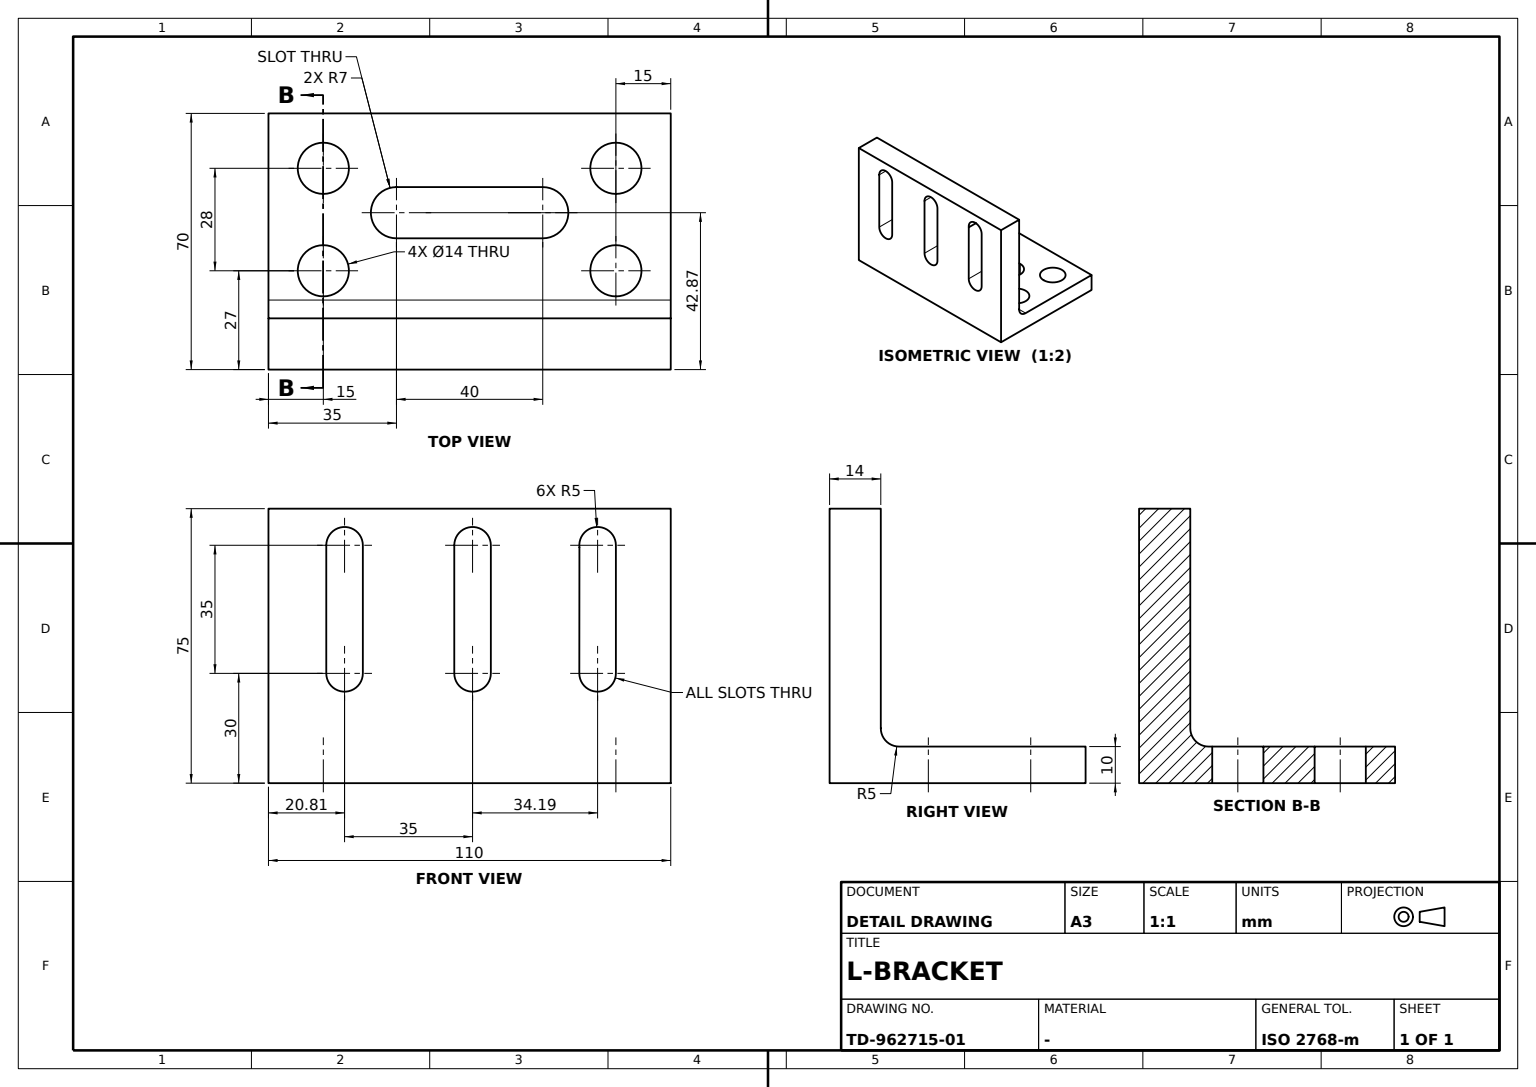
ISO-10303-21;
HEADER;
FILE_DESCRIPTION((''),'2;1');
FILE_NAME('','',(''),(''),'','','');
FILE_SCHEMA(('AUTOMOTIVE_DESIGN'));
ENDSEC;
DATA;
#1=APPLICATION_CONTEXT('');
#2=PRODUCT_CONTEXT('',#1,'mechanical');
#3=PRODUCT('','','',(#2));
#4=PRODUCT_DEFINITION_FORMATION('','',#3);
#5=PRODUCT_DEFINITION_CONTEXT('',#1,'design');
#6=PRODUCT_DEFINITION('','',#4,#5);
#7=PRODUCT_DEFINITION_SHAPE('','',#6);
#8=(LENGTH_UNIT()NAMED_UNIT(*)SI_UNIT(.MILLI.,.METRE.));
#9=(NAMED_UNIT(*)PLANE_ANGLE_UNIT()SI_UNIT($,.RADIAN.));
#10=(NAMED_UNIT(*)SI_UNIT($,.STERADIAN.)SOLID_ANGLE_UNIT());
#11=UNCERTAINTY_MEASURE_WITH_UNIT(LENGTH_MEASURE(0.005),#8,'distance_accuracy_value','');
#12=(GEOMETRIC_REPRESENTATION_CONTEXT(3)GLOBAL_UNCERTAINTY_ASSIGNED_CONTEXT((#11))GLOBAL_UNIT_ASSIGNED_CONTEXT((#8,#9,#10))REPRESENTATION_CONTEXT('',''));
#13=CARTESIAN_POINT('',(-7.,-24.969351,44.348961));
#14=VERTEX_POINT('',#13);
#15=CARTESIAN_POINT('',(7.,-24.969351,44.348961));
#16=VERTEX_POINT('',#15);
#17=DIRECTION('',(-1.,0.,0.));
#18=VECTOR('',#17,1000.);
#19=LINE('',#13,#18);
#20=EDGE_CURVE('',#14,#16,#19,.F.);
#21=ORIENTED_EDGE('',*,*,#20,.T.);
#22=CARTESIAN_POINT('',(7.,-24.999998,9.906179));
#23=VERTEX_POINT('',#22);
#24=CARTESIAN_POINT('',(7.,-25.026676,-20.076002));
#25=DIRECTION('',(0.,-0.000889801,-0.999999604));
#26=VECTOR('',#25,1000.);
#27=LINE('',#24,#26);
#28=EDGE_CURVE('',#16,#23,#27,.T.);
#29=ORIENTED_EDGE('',*,*,#28,.T.);
#30=CARTESIAN_POINT('',(-7.,-24.999998,9.906179));
#31=VERTEX_POINT('',#30);
#32=CARTESIAN_POINT('',(0.66,-24.999998,9.906179));
#33=LINE('',#32,#18);
#34=EDGE_CURVE('',#31,#23,#33,.F.);
#35=ORIENTED_EDGE('',*,*,#34,.F.);
#36=LINE('',#13,#26);
#37=EDGE_CURVE('',#14,#31,#36,.T.);
#38=ORIENTED_EDGE('',*,*,#37,.F.);
#39=EDGE_LOOP('',(#21,#29,#35,#38));
#40=FACE_BOUND('',#39,.T.);
#41=DIRECTION('',(0.,-0.999999604,0.000889801));
#42=AXIS2_PLACEMENT_3D('',#13,#41,#25);
#43=PLANE('',#42);
#44=ADVANCED_FACE('',(#40),#43,.F.);
#45=CARTESIAN_POINT('',(-7.,-15.,9.90173));
#46=VERTEX_POINT('',#45);
#47=CARTESIAN_POINT('',(-7.,-20.,9.90173));
#48=DIRECTION('',(0.,0.,1.));
#49=AXIS2_PLACEMENT_3D('',#47,#17,#48);
#50=CIRCLE('',#49,5.);
#51=EDGE_CURVE('',#46,#31,#50,.T.);
#52=ORIENTED_EDGE('',*,*,#51,.T.);
#53=ORIENTED_EDGE('',*,*,#34,.T.);
#54=CARTESIAN_POINT('',(7.,-15.,9.90173));
#55=VERTEX_POINT('',#54);
#56=CARTESIAN_POINT('',(7.,-20.,9.90173));
#57=DIRECTION('',(1.,0.,0.));
#58=DIRECTION('',(0.,0.,-1.));
#59=AXIS2_PLACEMENT_3D('',#56,#57,#58);
#60=CIRCLE('',#59,5.);
#61=EDGE_CURVE('',#23,#55,#60,.T.);
#62=ORIENTED_EDGE('',*,*,#61,.T.);
#63=CARTESIAN_POINT('',(0.66,-15.,9.90173));
#64=LINE('',#63,#18);
#65=EDGE_CURVE('',#46,#55,#64,.F.);
#66=ORIENTED_EDGE('',*,*,#65,.F.);
#67=EDGE_LOOP('',(#52,#53,#62,#66));
#68=FACE_BOUND('',#67,.T.);
#69=CARTESIAN_POINT('',(0.66,-20.,9.90173));
#70=DIRECTION('',(0.,-1.,0.));
#71=AXIS2_PLACEMENT_3D('',#69,#17,#70);
#72=CYLINDRICAL_SURFACE('',#71,5.);
#73=ADVANCED_FACE('',(#68),#72,.F.);
#74=CARTESIAN_POINT('',(-28.867531,-35.,-20.09827));
#75=VERTEX_POINT('',#74);
#76=CARTESIAN_POINT('',(-28.867531,-75.,-20.09827));
#77=VERTEX_POINT('',#76);
#78=CARTESIAN_POINT('',(-28.867531,0.,-20.09827));
#79=VECTOR('',#70,1000.);
#80=LINE('',#78,#79);
#81=EDGE_CURVE('',#75,#77,#80,.T.);
#82=ORIENTED_EDGE('',*,*,#81,.T.);
#83=CARTESIAN_POINT('',(-28.867531,-75.,-10.09827));
#84=VERTEX_POINT('',#83);
#85=CARTESIAN_POINT('',(-28.867531,-75.,-15.75827));
#86=VECTOR('',#48,1000.);
#87=LINE('',#85,#86);
#88=EDGE_CURVE('',#84,#77,#87,.F.);
#89=ORIENTED_EDGE('',*,*,#88,.F.);
#90=CARTESIAN_POINT('',(-28.867531,-35.,-10.09827));
#91=VERTEX_POINT('',#90);
#92=LINE('',#90,#79);
#93=EDGE_CURVE('',#91,#84,#92,.T.);
#94=ORIENTED_EDGE('',*,*,#93,.F.);
#95=CARTESIAN_POINT('',(-28.867531,-35.,-15.75827));
#96=LINE('',#95,#86);
#97=EDGE_CURVE('',#91,#75,#96,.F.);
#98=ORIENTED_EDGE('',*,*,#97,.T.);
#99=EDGE_LOOP('',(#82,#89,#94,#98));
#100=FACE_BOUND('',#99,.T.);
#101=AXIS2_PLACEMENT_3D('',#90,#57,#70);
#102=PLANE('',#101);
#103=ADVANCED_FACE('',(#100),#102,.F.);
#104=CARTESIAN_POINT('',(7.,-15.,44.90173));
#105=VERTEX_POINT('',#104);
#106=CARTESIAN_POINT('',(7.,-20.,44.90173));
#107=AXIS2_PLACEMENT_3D('',#106,#57,#58);
#108=CIRCLE('',#107,5.);
#109=EDGE_CURVE('',#105,#16,#108,.T.);
#110=ORIENTED_EDGE('',*,*,#109,.T.);
#111=ORIENTED_EDGE('',*,*,#20,.F.);
#112=CARTESIAN_POINT('',(-7.,-15.,44.90173));
#113=VERTEX_POINT('',#112);
#114=CARTESIAN_POINT('',(-7.,-20.,44.90173));
#115=AXIS2_PLACEMENT_3D('',#114,#17,#48);
#116=CIRCLE('',#115,5.);
#117=EDGE_CURVE('',#14,#113,#116,.T.);
#118=ORIENTED_EDGE('',*,*,#117,.T.);
#119=CARTESIAN_POINT('',(0.66,-15.,44.90173));
#120=LINE('',#119,#18);
#121=EDGE_CURVE('',#113,#105,#120,.F.);
#122=ORIENTED_EDGE('',*,*,#121,.T.);
#123=EDGE_LOOP('',(#110,#111,#118,#122));
#124=FACE_BOUND('',#123,.T.);
#125=CARTESIAN_POINT('',(0.66,-20.,44.90173));
#126=AXIS2_PLACEMENT_3D('',#125,#17,#70);
#127=CYLINDRICAL_SURFACE('',#126,5.);
#128=ADVANCED_FACE('',(#124),#127,.F.);
#129=VECTOR('',#58,1000.);
#130=LINE('',#112,#129);
#131=EDGE_CURVE('',#113,#46,#130,.T.);
#132=ORIENTED_EDGE('',*,*,#131,.T.);
#133=ORIENTED_EDGE('',*,*,#65,.T.);
#134=CARTESIAN_POINT('',(7.,-15.,-20.09827));
#135=LINE('',#134,#129);
#136=EDGE_CURVE('',#105,#55,#135,.T.);
#137=ORIENTED_EDGE('',*,*,#136,.F.);
#138=ORIENTED_EDGE('',*,*,#121,.F.);
#139=EDGE_LOOP('',(#132,#133,#137,#138));
#140=FACE_BOUND('',#139,.T.);
#141=AXIS2_PLACEMENT_3D('',#112,#70,#58);
#142=PLANE('',#141);
#143=ADVANCED_FACE('',(#140),#142,.T.);
#144=CARTESIAN_POINT('',(-13.,-15.,-10.09827));
#145=VERTEX_POINT('',#144);
#146=CARTESIAN_POINT('',(-20.,-15.,-10.09827));
#147=AXIS2_PLACEMENT_3D('',#146,#48,#57);
#148=CIRCLE('',#147,7.);
#149=EDGE_CURVE('',#145,#145,#148,.T.);
#150=ORIENTED_EDGE('',*,*,#149,.T.);
#151=EDGE_LOOP('',(#150));
#152=FACE_BOUND('',#151,.T.);
#153=CARTESIAN_POINT('',(-27.,-15.,-20.09827));
#154=VERTEX_POINT('',#153);
#155=CARTESIAN_POINT('',(-20.,-15.,-20.09827));
#156=AXIS2_PLACEMENT_3D('',#155,#58,#17);
#157=CIRCLE('',#156,7.);
#158=EDGE_CURVE('',#154,#154,#157,.T.);
#159=ORIENTED_EDGE('',*,*,#158,.T.);
#160=EDGE_LOOP('',(#159));
#161=FACE_BOUND('',#160,.T.);
#162=CARTESIAN_POINT('',(-20.,-15.,-15.75827));
#163=AXIS2_PLACEMENT_3D('',#162,#48,#57);
#164=CYLINDRICAL_SURFACE('',#163,7.);
#165=ADVANCED_FACE('',(#152,#161),#164,.F.);
#166=CARTESIAN_POINT('',(7.,-84.190727,44.90173));
#167=VERTEX_POINT('',#166);
#168=CARTESIAN_POINT('',(7.,-94.190727,44.90173));
#169=VERTEX_POINT('',#168);
#170=CARTESIAN_POINT('',(7.,-89.190727,44.90173));
#171=AXIS2_PLACEMENT_3D('',#170,#57,#58);
#172=CIRCLE('',#171,5.);
#173=EDGE_CURVE('',#167,#169,#172,.T.);
#174=ORIENTED_EDGE('',*,*,#173,.F.);
#175=CARTESIAN_POINT('',(7.,-84.190727,9.90173));
#176=VERTEX_POINT('',#175);
#177=CARTESIAN_POINT('',(7.,-84.190727,-20.09827));
#178=LINE('',#177,#129);
#179=EDGE_CURVE('',#167,#176,#178,.T.);
#180=ORIENTED_EDGE('',*,*,#179,.T.);
#181=CARTESIAN_POINT('',(7.,-94.190727,9.90173));
#182=VERTEX_POINT('',#181);
#183=CARTESIAN_POINT('',(7.,-89.190727,9.90173));
#184=AXIS2_PLACEMENT_3D('',#183,#57,#58);
#185=CIRCLE('',#184,5.);
#186=EDGE_CURVE('',#182,#176,#185,.T.);
#187=ORIENTED_EDGE('',*,*,#186,.F.);
#188=CARTESIAN_POINT('',(7.,-94.190727,-20.09827));
#189=LINE('',#188,#129);
#190=EDGE_CURVE('',#169,#182,#189,.T.);
#191=ORIENTED_EDGE('',*,*,#190,.F.);
#192=EDGE_LOOP('',(#174,#180,#187,#191));
#193=FACE_BOUND('',#192,.T.);
#194=ORIENTED_EDGE('',*,*,#61,.F.);
#195=ORIENTED_EDGE('',*,*,#28,.F.);
#196=ORIENTED_EDGE('',*,*,#109,.F.);
#197=ORIENTED_EDGE('',*,*,#136,.T.);
#198=EDGE_LOOP('',(#194,#195,#196,#197));
#199=FACE_BOUND('',#198,.T.);
#200=CARTESIAN_POINT('',(7.,-59.190727,44.90173));
#201=VERTEX_POINT('',#200);
#202=CARTESIAN_POINT('',(7.,-59.190727,9.90173));
#203=VERTEX_POINT('',#202);
#204=CARTESIAN_POINT('',(7.,-59.190727,-20.09827));
#205=LINE('',#204,#129);
#206=EDGE_CURVE('',#201,#203,#205,.T.);
#207=ORIENTED_EDGE('',*,*,#206,.F.);
#208=CARTESIAN_POINT('',(7.,-49.190727,44.90173));
#209=VERTEX_POINT('',#208);
#210=CARTESIAN_POINT('',(7.,-54.190727,44.90173));
#211=AXIS2_PLACEMENT_3D('',#210,#57,#58);
#212=CIRCLE('',#211,5.);
#213=EDGE_CURVE('',#209,#201,#212,.T.);
#214=ORIENTED_EDGE('',*,*,#213,.F.);
#215=CARTESIAN_POINT('',(7.,-49.190727,9.90173));
#216=VERTEX_POINT('',#215);
#217=CARTESIAN_POINT('',(7.,-49.190727,-20.09827));
#218=LINE('',#217,#129);
#219=EDGE_CURVE('',#209,#216,#218,.T.);
#220=ORIENTED_EDGE('',*,*,#219,.T.);
#221=CARTESIAN_POINT('',(7.,-54.190727,9.90173));
#222=AXIS2_PLACEMENT_3D('',#221,#57,#58);
#223=CIRCLE('',#222,5.);
#224=EDGE_CURVE('',#203,#216,#223,.T.);
#225=ORIENTED_EDGE('',*,*,#224,.F.);
#226=EDGE_LOOP('',(#207,#214,#220,#225));
#227=FACE_BOUND('',#226,.T.);
#228=CARTESIAN_POINT('',(7.,0.,54.90173));
#229=VERTEX_POINT('',#228);
#230=CARTESIAN_POINT('',(7.,-110.,54.90173));
#231=VERTEX_POINT('',#230);
#232=LINE('',#228,#79);
#233=EDGE_CURVE('',#229,#231,#232,.T.);
#234=ORIENTED_EDGE('',*,*,#233,.T.);
#235=CARTESIAN_POINT('',(7.,-110.,-20.09827));
#236=VERTEX_POINT('',#235);
#237=LINE('',#235,#86);
#238=EDGE_CURVE('',#236,#231,#237,.T.);
#239=ORIENTED_EDGE('',*,*,#238,.F.);
#240=CARTESIAN_POINT('',(7.,0.,-20.09827));
#241=VERTEX_POINT('',#240);
#242=LINE('',#240,#79);
#243=EDGE_CURVE('',#241,#236,#242,.T.);
#244=ORIENTED_EDGE('',*,*,#243,.F.);
#245=LINE('',#240,#86);
#246=EDGE_CURVE('',#241,#229,#245,.T.);
#247=ORIENTED_EDGE('',*,*,#246,.T.);
#248=EDGE_LOOP('',(#234,#239,#244,#247));
#249=FACE_BOUND('',#248,.T.);
#250=AXIS2_PLACEMENT_3D('',#240,#57,#48);
#251=PLANE('',#250);
#252=ADVANCED_FACE('',(#193,#199,#227,#249),#251,.T.);
#253=CARTESIAN_POINT('',(-7.,-84.190727,9.90173));
#254=VERTEX_POINT('',#253);
#255=CARTESIAN_POINT('',(0.66,-84.190727,9.90173));
#256=LINE('',#255,#18);
#257=EDGE_CURVE('',#254,#176,#256,.F.);
#258=ORIENTED_EDGE('',*,*,#257,.F.);
#259=CARTESIAN_POINT('',(-7.,-94.190727,9.90173));
#260=VERTEX_POINT('',#259);
#261=CARTESIAN_POINT('',(-7.,-89.190727,9.90173));
#262=AXIS2_PLACEMENT_3D('',#261,#17,#48);
#263=CIRCLE('',#262,5.);
#264=EDGE_CURVE('',#254,#260,#263,.T.);
#265=ORIENTED_EDGE('',*,*,#264,.T.);
#266=CARTESIAN_POINT('',(0.66,-94.190727,9.90173));
#267=LINE('',#266,#18);
#268=EDGE_CURVE('',#260,#182,#267,.F.);
#269=ORIENTED_EDGE('',*,*,#268,.T.);
#270=ORIENTED_EDGE('',*,*,#186,.T.);
#271=EDGE_LOOP('',(#258,#265,#269,#270));
#272=FACE_BOUND('',#271,.T.);
#273=CARTESIAN_POINT('',(0.66,-89.190727,9.90173));
#274=AXIS2_PLACEMENT_3D('',#273,#17,#70);
#275=CYLINDRICAL_SURFACE('',#274,5.);
#276=ADVANCED_FACE('',(#272),#275,.F.);
#277=CARTESIAN_POINT('',(-27.,-95.,-20.09827));
#278=VERTEX_POINT('',#277);
#279=CARTESIAN_POINT('',(-20.,-95.,-20.09827));
#280=AXIS2_PLACEMENT_3D('',#279,#58,#17);
#281=CIRCLE('',#280,7.);
#282=EDGE_CURVE('',#278,#278,#281,.T.);
#283=ORIENTED_EDGE('',*,*,#282,.F.);
#284=EDGE_LOOP('',(#283));
#285=FACE_BOUND('',#284,.T.);
#286=ORIENTED_EDGE('',*,*,#158,.F.);
#287=EDGE_LOOP('',(#286));
#288=FACE_BOUND('',#287,.T.);
#289=CARTESIAN_POINT('',(-63.,0.,-20.09827));
#290=VERTEX_POINT('',#289);
#291=CARTESIAN_POINT('',(-63.,-110.,-20.09827));
#292=VERTEX_POINT('',#291);
#293=LINE('',#289,#79);
#294=EDGE_CURVE('',#290,#292,#293,.T.);
#295=ORIENTED_EDGE('',*,*,#294,.F.);
#296=VECTOR('',#57,1000.);
#297=LINE('',#289,#296);
#298=EDGE_CURVE('',#290,#241,#297,.T.);
#299=ORIENTED_EDGE('',*,*,#298,.T.);
#300=ORIENTED_EDGE('',*,*,#243,.T.);
#301=LINE('',#291,#296);
#302=EDGE_CURVE('',#292,#236,#301,.T.);
#303=ORIENTED_EDGE('',*,*,#302,.F.);
#304=EDGE_LOOP('',(#295,#299,#300,#303));
#305=FACE_BOUND('',#304,.T.);
#306=CARTESIAN_POINT('',(-55.,-15.,-20.09827));
#307=VERTEX_POINT('',#306);
#308=CARTESIAN_POINT('',(-48.,-15.,-20.09827));
#309=AXIS2_PLACEMENT_3D('',#308,#58,#17);
#310=CIRCLE('',#309,7.);
#311=EDGE_CURVE('',#307,#307,#310,.T.);
#312=ORIENTED_EDGE('',*,*,#311,.F.);
#313=EDGE_LOOP('',(#312));
#314=FACE_BOUND('',#313,.T.);
#315=CARTESIAN_POINT('',(-42.867531,-75.,-20.09827));
#316=VERTEX_POINT('',#315);
#317=CARTESIAN_POINT('',(-35.867531,-75.,-20.09827));
#318=AXIS2_PLACEMENT_3D('',#317,#58,#17);
#319=CIRCLE('',#318,7.);
#320=EDGE_CURVE('',#77,#316,#319,.T.);
#321=ORIENTED_EDGE('',*,*,#320,.F.);
#322=ORIENTED_EDGE('',*,*,#81,.F.);
#323=CARTESIAN_POINT('',(-42.867531,-35.,-20.09827));
#324=VERTEX_POINT('',#323);
#325=CARTESIAN_POINT('',(-35.867531,-35.,-20.09827));
#326=AXIS2_PLACEMENT_3D('',#325,#58,#17);
#327=CIRCLE('',#326,7.);
#328=EDGE_CURVE('',#324,#75,#327,.T.);
#329=ORIENTED_EDGE('',*,*,#328,.F.);
#330=CARTESIAN_POINT('',(-42.867531,0.,-20.09827));
#331=LINE('',#330,#79);
#332=EDGE_CURVE('',#324,#316,#331,.T.);
#333=ORIENTED_EDGE('',*,*,#332,.T.);
#334=EDGE_LOOP('',(#321,#322,#329,#333));
#335=FACE_BOUND('',#334,.T.);
#336=CARTESIAN_POINT('',(-55.,-95.,-20.09827));
#337=VERTEX_POINT('',#336);
#338=CARTESIAN_POINT('',(-48.,-95.,-20.09827));
#339=AXIS2_PLACEMENT_3D('',#338,#58,#17);
#340=CIRCLE('',#339,7.);
#341=EDGE_CURVE('',#337,#337,#340,.T.);
#342=ORIENTED_EDGE('',*,*,#341,.F.);
#343=EDGE_LOOP('',(#342));
#344=FACE_BOUND('',#343,.T.);
#345=AXIS2_PLACEMENT_3D('',#289,#58,#57);
#346=PLANE('',#345);
#347=ADVANCED_FACE('',(#285,#288,#305,#314,#335,#344),#346,.T.);
#348=CARTESIAN_POINT('',(-42.867531,-35.,-10.09827));
#349=VERTEX_POINT('',#348);
#350=CARTESIAN_POINT('',(-42.867531,-35.,-15.75827));
#351=LINE('',#350,#86);
#352=EDGE_CURVE('',#349,#324,#351,.F.);
#353=ORIENTED_EDGE('',*,*,#352,.F.);
#354=CARTESIAN_POINT('',(-42.867531,-75.,-10.09827));
#355=VERTEX_POINT('',#354);
#356=LINE('',#348,#79);
#357=EDGE_CURVE('',#349,#355,#356,.T.);
#358=ORIENTED_EDGE('',*,*,#357,.T.);
#359=CARTESIAN_POINT('',(-42.867531,-75.,-15.75827));
#360=LINE('',#359,#86);
#361=EDGE_CURVE('',#355,#316,#360,.F.);
#362=ORIENTED_EDGE('',*,*,#361,.T.);
#363=ORIENTED_EDGE('',*,*,#332,.F.);
#364=EDGE_LOOP('',(#353,#358,#362,#363));
#365=FACE_BOUND('',#364,.T.);
#366=AXIS2_PLACEMENT_3D('',#348,#57,#70);
#367=PLANE('',#366);
#368=ADVANCED_FACE('',(#365),#367,.T.);
#369=ORIENTED_EDGE('',*,*,#233,.F.);
#370=CARTESIAN_POINT('',(-7.,0.,54.90173));
#371=VERTEX_POINT('',#370);
#372=LINE('',#228,#18);
#373=EDGE_CURVE('',#229,#371,#372,.T.);
#374=ORIENTED_EDGE('',*,*,#373,.T.);
#375=CARTESIAN_POINT('',(-7.,-110.,54.90173));
#376=VERTEX_POINT('',#375);
#377=LINE('',#370,#79);
#378=EDGE_CURVE('',#371,#376,#377,.T.);
#379=ORIENTED_EDGE('',*,*,#378,.T.);
#380=LINE('',#230,#18);
#381=EDGE_CURVE('',#231,#376,#380,.T.);
#382=ORIENTED_EDGE('',*,*,#381,.F.);
#383=EDGE_LOOP('',(#369,#374,#379,#382));
#384=FACE_BOUND('',#383,.T.);
#385=AXIS2_PLACEMENT_3D('',#228,#48,#17);
#386=PLANE('',#385);
#387=ADVANCED_FACE('',(#384),#386,.T.);
#388=CARTESIAN_POINT('',(-7.,-49.190727,9.90173));
#389=VERTEX_POINT('',#388);
#390=CARTESIAN_POINT('',(0.66,-49.190727,9.90173));
#391=LINE('',#390,#18);
#392=EDGE_CURVE('',#389,#216,#391,.F.);
#393=ORIENTED_EDGE('',*,*,#392,.T.);
#394=ORIENTED_EDGE('',*,*,#219,.F.);
#395=CARTESIAN_POINT('',(-7.,-49.190727,44.90173));
#396=VERTEX_POINT('',#395);
#397=CARTESIAN_POINT('',(0.66,-49.190727,44.90173));
#398=LINE('',#397,#18);
#399=EDGE_CURVE('',#396,#209,#398,.F.);
#400=ORIENTED_EDGE('',*,*,#399,.F.);
#401=LINE('',#395,#129);
#402=EDGE_CURVE('',#396,#389,#401,.T.);
#403=ORIENTED_EDGE('',*,*,#402,.T.);
#404=EDGE_LOOP('',(#393,#394,#400,#403));
#405=FACE_BOUND('',#404,.T.);
#406=AXIS2_PLACEMENT_3D('',#395,#70,#58);
#407=PLANE('',#406);
#408=ADVANCED_FACE('',(#405),#407,.T.);
#409=CARTESIAN_POINT('',(-7.,-59.190727,44.90173));
#410=VERTEX_POINT('',#409);
#411=CARTESIAN_POINT('',(0.66,-59.190727,44.90173));
#412=LINE('',#411,#18);
#413=EDGE_CURVE('',#410,#201,#412,.F.);
#414=ORIENTED_EDGE('',*,*,#413,.T.);
#415=ORIENTED_EDGE('',*,*,#206,.T.);
#416=CARTESIAN_POINT('',(-7.,-59.190727,9.90173));
#417=VERTEX_POINT('',#416);
#418=CARTESIAN_POINT('',(0.66,-59.190727,9.90173));
#419=LINE('',#418,#18);
#420=EDGE_CURVE('',#417,#203,#419,.F.);
#421=ORIENTED_EDGE('',*,*,#420,.F.);
#422=LINE('',#409,#129);
#423=EDGE_CURVE('',#410,#417,#422,.T.);
#424=ORIENTED_EDGE('',*,*,#423,.F.);
#425=EDGE_LOOP('',(#414,#415,#421,#424));
#426=FACE_BOUND('',#425,.T.);
#427=AXIS2_PLACEMENT_3D('',#409,#70,#58);
#428=PLANE('',#427);
#429=ADVANCED_FACE('',(#426),#428,.F.);
#430=ORIENTED_EDGE('',*,*,#341,.T.);
#431=EDGE_LOOP('',(#430));
#432=FACE_BOUND('',#431,.T.);
#433=CARTESIAN_POINT('',(-41.,-95.,-10.09827));
#434=VERTEX_POINT('',#433);
#435=CARTESIAN_POINT('',(-48.,-95.,-10.09827));
#436=AXIS2_PLACEMENT_3D('',#435,#48,#57);
#437=CIRCLE('',#436,7.);
#438=EDGE_CURVE('',#434,#434,#437,.T.);
#439=ORIENTED_EDGE('',*,*,#438,.T.);
#440=EDGE_LOOP('',(#439));
#441=FACE_BOUND('',#440,.T.);
#442=CARTESIAN_POINT('',(-48.,-95.,-15.75827));
#443=AXIS2_PLACEMENT_3D('',#442,#48,#57);
#444=CYLINDRICAL_SURFACE('',#443,7.);
#445=ADVANCED_FACE('',(#432,#441),#444,.F.);
#446=CARTESIAN_POINT('',(-35.867531,-75.,-10.09827));
#447=AXIS2_PLACEMENT_3D('',#446,#48,#57);
#448=CIRCLE('',#447,7.);
#449=EDGE_CURVE('',#355,#84,#448,.T.);
#450=ORIENTED_EDGE('',*,*,#449,.T.);
#451=ORIENTED_EDGE('',*,*,#88,.T.);
#452=ORIENTED_EDGE('',*,*,#320,.T.);
#453=ORIENTED_EDGE('',*,*,#361,.F.);
#454=EDGE_LOOP('',(#450,#451,#452,#453));
#455=FACE_BOUND('',#454,.T.);
#456=CARTESIAN_POINT('',(-35.867531,-75.,-15.75827));
#457=AXIS2_PLACEMENT_3D('',#456,#48,#57);
#458=CYLINDRICAL_SURFACE('',#457,7.);
#459=ADVANCED_FACE('',(#455),#458,.F.);
#460=ORIENTED_EDGE('',*,*,#246,.F.);
#461=ORIENTED_EDGE('',*,*,#298,.F.);
#462=CARTESIAN_POINT('',(-63.,0.,-10.09827));
#463=VERTEX_POINT('',#462);
#464=LINE('',#462,#129);
#465=EDGE_CURVE('',#463,#290,#464,.T.);
#466=ORIENTED_EDGE('',*,*,#465,.F.);
#467=CARTESIAN_POINT('',(-12.,0.,-10.09827));
#468=VERTEX_POINT('',#467);
#469=CARTESIAN_POINT('',(-7.,0.,-10.09827));
#470=LINE('',#469,#18);
#471=EDGE_CURVE('',#468,#463,#470,.T.);
#472=ORIENTED_EDGE('',*,*,#471,.F.);
#473=CARTESIAN_POINT('',(-7.,0.,-5.09827));
#474=VERTEX_POINT('',#473);
#475=CARTESIAN_POINT('',(-12.,0.,-5.09827));
#476=DIRECTION('',(0.,1.,0.));
#477=AXIS2_PLACEMENT_3D('',#475,#476,#48);
#478=CIRCLE('',#477,5.);
#479=EDGE_CURVE('',#474,#468,#478,.T.);
#480=ORIENTED_EDGE('',*,*,#479,.F.);
#481=LINE('',#370,#129);
#482=EDGE_CURVE('',#371,#474,#481,.T.);
#483=ORIENTED_EDGE('',*,*,#482,.F.);
#484=ORIENTED_EDGE('',*,*,#373,.F.);
#485=EDGE_LOOP('',(#460,#461,#466,#472,#480,#483,#484));
#486=FACE_BOUND('',#485,.T.);
#487=CARTESIAN_POINT('',(0.,0.,0.));
#488=AXIS2_PLACEMENT_3D('',#487,#476,#17);
#489=PLANE('',#488);
#490=ADVANCED_FACE('',(#486),#489,.T.);
#491=CARTESIAN_POINT('',(-41.,-15.,-10.09827));
#492=VERTEX_POINT('',#491);
#493=CARTESIAN_POINT('',(-48.,-15.,-10.09827));
#494=AXIS2_PLACEMENT_3D('',#493,#48,#57);
#495=CIRCLE('',#494,7.);
#496=EDGE_CURVE('',#492,#492,#495,.T.);
#497=ORIENTED_EDGE('',*,*,#496,.F.);
#498=EDGE_LOOP('',(#497));
#499=FACE_BOUND('',#498,.T.);
#500=ORIENTED_EDGE('',*,*,#149,.F.);
#501=EDGE_LOOP('',(#500));
#502=FACE_BOUND('',#501,.T.);
#503=ORIENTED_EDGE('',*,*,#449,.F.);
#504=ORIENTED_EDGE('',*,*,#357,.F.);
#505=CARTESIAN_POINT('',(-35.867531,-35.,-10.09827));
#506=AXIS2_PLACEMENT_3D('',#505,#48,#57);
#507=CIRCLE('',#506,7.);
#508=EDGE_CURVE('',#91,#349,#507,.T.);
#509=ORIENTED_EDGE('',*,*,#508,.F.);
#510=ORIENTED_EDGE('',*,*,#93,.T.);
#511=EDGE_LOOP('',(#503,#504,#509,#510));
#512=FACE_BOUND('',#511,.T.);
#513=CARTESIAN_POINT('',(-13.,-95.,-10.09827));
#514=VERTEX_POINT('',#513);
#515=CARTESIAN_POINT('',(-20.,-95.,-10.09827));
#516=AXIS2_PLACEMENT_3D('',#515,#48,#57);
#517=CIRCLE('',#516,7.);
#518=EDGE_CURVE('',#514,#514,#517,.T.);
#519=ORIENTED_EDGE('',*,*,#518,.F.);
#520=EDGE_LOOP('',(#519));
#521=FACE_BOUND('',#520,.T.);
#522=ORIENTED_EDGE('',*,*,#438,.F.);
#523=EDGE_LOOP('',(#522));
#524=FACE_BOUND('',#523,.T.);
#525=ORIENTED_EDGE('',*,*,#471,.T.);
#526=CARTESIAN_POINT('',(-63.,-110.,-10.09827));
#527=VERTEX_POINT('',#526);
#528=LINE('',#462,#79);
#529=EDGE_CURVE('',#463,#527,#528,.T.);
#530=ORIENTED_EDGE('',*,*,#529,.T.);
#531=CARTESIAN_POINT('',(-12.,-110.,-10.09827));
#532=VERTEX_POINT('',#531);
#533=CARTESIAN_POINT('',(-7.,-110.,-10.09827));
#534=LINE('',#533,#18);
#535=EDGE_CURVE('',#532,#527,#534,.T.);
#536=ORIENTED_EDGE('',*,*,#535,.F.);
#537=CARTESIAN_POINT('',(-12.,-55.,-10.09827));
#538=LINE('',#537,#79);
#539=EDGE_CURVE('',#468,#532,#538,.T.);
#540=ORIENTED_EDGE('',*,*,#539,.F.);
#541=EDGE_LOOP('',(#525,#530,#536,#540));
#542=FACE_BOUND('',#541,.T.);
#543=AXIS2_PLACEMENT_3D('',#469,#48,#17);
#544=PLANE('',#543);
#545=ADVANCED_FACE('',(#499,#502,#512,#521,#524,#542),#544,.T.);
#546=CARTESIAN_POINT('',(-7.,-94.190727,44.90173));
#547=VERTEX_POINT('',#546);
#548=CARTESIAN_POINT('',(0.66,-94.190727,44.90173));
#549=LINE('',#548,#18);
#550=EDGE_CURVE('',#547,#169,#549,.F.);
#551=ORIENTED_EDGE('',*,*,#550,.T.);
#552=ORIENTED_EDGE('',*,*,#190,.T.);
#553=ORIENTED_EDGE('',*,*,#268,.F.);
#554=LINE('',#546,#129);
#555=EDGE_CURVE('',#547,#260,#554,.T.);
#556=ORIENTED_EDGE('',*,*,#555,.F.);
#557=EDGE_LOOP('',(#551,#552,#553,#556));
#558=FACE_BOUND('',#557,.T.);
#559=AXIS2_PLACEMENT_3D('',#546,#70,#58);
#560=PLANE('',#559);
#561=ADVANCED_FACE('',(#558),#560,.F.);
#562=ORIENTED_EDGE('',*,*,#550,.F.);
#563=CARTESIAN_POINT('',(-7.,-84.190727,44.90173));
#564=VERTEX_POINT('',#563);
#565=CARTESIAN_POINT('',(-7.,-89.190727,44.90173));
#566=AXIS2_PLACEMENT_3D('',#565,#17,#48);
#567=CIRCLE('',#566,5.);
#568=EDGE_CURVE('',#547,#564,#567,.T.);
#569=ORIENTED_EDGE('',*,*,#568,.T.);
#570=CARTESIAN_POINT('',(0.66,-84.190727,44.90173));
#571=LINE('',#570,#18);
#572=EDGE_CURVE('',#564,#167,#571,.F.);
#573=ORIENTED_EDGE('',*,*,#572,.T.);
#574=ORIENTED_EDGE('',*,*,#173,.T.);
#575=EDGE_LOOP('',(#562,#569,#573,#574));
#576=FACE_BOUND('',#575,.T.);
#577=CARTESIAN_POINT('',(0.66,-89.190727,44.90173));
#578=AXIS2_PLACEMENT_3D('',#577,#17,#70);
#579=CYLINDRICAL_SURFACE('',#578,5.);
#580=ADVANCED_FACE('',(#576),#579,.F.);
#581=ORIENTED_EDGE('',*,*,#282,.T.);
#582=EDGE_LOOP('',(#581));
#583=FACE_BOUND('',#582,.T.);
#584=ORIENTED_EDGE('',*,*,#518,.T.);
#585=EDGE_LOOP('',(#584));
#586=FACE_BOUND('',#585,.T.);
#587=CARTESIAN_POINT('',(-20.,-95.,-15.75827));
#588=AXIS2_PLACEMENT_3D('',#587,#48,#57);
#589=CYLINDRICAL_SURFACE('',#588,7.);
#590=ADVANCED_FACE('',(#583,#586),#589,.F.);
#591=ORIENTED_EDGE('',*,*,#392,.F.);
#592=CARTESIAN_POINT('',(-7.,-54.190727,9.90173));
#593=AXIS2_PLACEMENT_3D('',#592,#17,#48);
#594=CIRCLE('',#593,5.);
#595=EDGE_CURVE('',#389,#417,#594,.T.);
#596=ORIENTED_EDGE('',*,*,#595,.T.);
#597=ORIENTED_EDGE('',*,*,#420,.T.);
#598=ORIENTED_EDGE('',*,*,#224,.T.);
#599=EDGE_LOOP('',(#591,#596,#597,#598));
#600=FACE_BOUND('',#599,.T.);
#601=CARTESIAN_POINT('',(0.66,-54.190727,9.90173));
#602=AXIS2_PLACEMENT_3D('',#601,#17,#70);
#603=CYLINDRICAL_SURFACE('',#602,5.);
#604=ADVANCED_FACE('',(#600),#603,.F.);
#605=ORIENTED_EDGE('',*,*,#496,.T.);
#606=EDGE_LOOP('',(#605));
#607=FACE_BOUND('',#606,.T.);
#608=ORIENTED_EDGE('',*,*,#311,.T.);
#609=EDGE_LOOP('',(#608));
#610=FACE_BOUND('',#609,.T.);
#611=CARTESIAN_POINT('',(-48.,-15.,-15.75827));
#612=AXIS2_PLACEMENT_3D('',#611,#48,#57);
#613=CYLINDRICAL_SURFACE('',#612,7.);
#614=ADVANCED_FACE('',(#607,#610),#613,.F.);
#615=ORIENTED_EDGE('',*,*,#51,.F.);
#616=ORIENTED_EDGE('',*,*,#131,.F.);
#617=ORIENTED_EDGE('',*,*,#117,.F.);
#618=ORIENTED_EDGE('',*,*,#37,.T.);
#619=EDGE_LOOP('',(#615,#616,#617,#618));
#620=FACE_BOUND('',#619,.T.);
#621=ORIENTED_EDGE('',*,*,#423,.T.);
#622=ORIENTED_EDGE('',*,*,#595,.F.);
#623=ORIENTED_EDGE('',*,*,#402,.F.);
#624=CARTESIAN_POINT('',(-7.,-54.190727,44.90173));
#625=AXIS2_PLACEMENT_3D('',#624,#17,#48);
#626=CIRCLE('',#625,5.);
#627=EDGE_CURVE('',#410,#396,#626,.T.);
#628=ORIENTED_EDGE('',*,*,#627,.F.);
#629=EDGE_LOOP('',(#621,#622,#623,#628));
#630=FACE_BOUND('',#629,.T.);
#631=ORIENTED_EDGE('',*,*,#378,.F.);
#632=ORIENTED_EDGE('',*,*,#482,.T.);
#633=CARTESIAN_POINT('',(-7.,-110.,-5.09827));
#634=VERTEX_POINT('',#633);
#635=CARTESIAN_POINT('',(-7.,-55.,-5.09827));
#636=LINE('',#635,#79);
#637=EDGE_CURVE('',#474,#634,#636,.T.);
#638=ORIENTED_EDGE('',*,*,#637,.T.);
#639=LINE('',#375,#129);
#640=EDGE_CURVE('',#376,#634,#639,.T.);
#641=ORIENTED_EDGE('',*,*,#640,.F.);
#642=EDGE_LOOP('',(#631,#632,#638,#641));
#643=FACE_BOUND('',#642,.T.);
#644=ORIENTED_EDGE('',*,*,#264,.F.);
#645=LINE('',#563,#129);
#646=EDGE_CURVE('',#564,#254,#645,.T.);
#647=ORIENTED_EDGE('',*,*,#646,.F.);
#648=ORIENTED_EDGE('',*,*,#568,.F.);
#649=ORIENTED_EDGE('',*,*,#555,.T.);
#650=EDGE_LOOP('',(#644,#647,#648,#649));
#651=FACE_BOUND('',#650,.T.);
#652=AXIS2_PLACEMENT_3D('',#370,#17,#58);
#653=PLANE('',#652);
#654=ADVANCED_FACE('',(#620,#630,#643,#651),#653,.T.);
#655=ORIENTED_EDGE('',*,*,#627,.T.);
#656=ORIENTED_EDGE('',*,*,#399,.T.);
#657=ORIENTED_EDGE('',*,*,#213,.T.);
#658=ORIENTED_EDGE('',*,*,#413,.F.);
#659=EDGE_LOOP('',(#655,#656,#657,#658));
#660=FACE_BOUND('',#659,.T.);
#661=CARTESIAN_POINT('',(0.66,-54.190727,44.90173));
#662=AXIS2_PLACEMENT_3D('',#661,#17,#70);
#663=CYLINDRICAL_SURFACE('',#662,5.);
#664=ADVANCED_FACE('',(#660),#663,.F.);
#665=ORIENTED_EDGE('',*,*,#352,.T.);
#666=ORIENTED_EDGE('',*,*,#328,.T.);
#667=ORIENTED_EDGE('',*,*,#97,.F.);
#668=ORIENTED_EDGE('',*,*,#508,.T.);
#669=EDGE_LOOP('',(#665,#666,#667,#668));
#670=FACE_BOUND('',#669,.T.);
#671=CARTESIAN_POINT('',(-35.867531,-35.,-15.75827));
#672=AXIS2_PLACEMENT_3D('',#671,#48,#57);
#673=CYLINDRICAL_SURFACE('',#672,7.);
#674=ADVANCED_FACE('',(#670),#673,.F.);
#675=ORIENTED_EDGE('',*,*,#539,.T.);
#676=CARTESIAN_POINT('',(-12.,-110.,-5.09827));
#677=AXIS2_PLACEMENT_3D('',#676,#476,#48);
#678=CIRCLE('',#677,5.);
#679=EDGE_CURVE('',#634,#532,#678,.T.);
#680=ORIENTED_EDGE('',*,*,#679,.F.);
#681=ORIENTED_EDGE('',*,*,#637,.F.);
#682=ORIENTED_EDGE('',*,*,#479,.T.);
#683=EDGE_LOOP('',(#675,#680,#681,#682));
#684=FACE_BOUND('',#683,.T.);
#685=CARTESIAN_POINT('',(-12.,-55.,-5.09827));
#686=AXIS2_PLACEMENT_3D('',#685,#70,#58);
#687=CYLINDRICAL_SURFACE('',#686,5.);
#688=ADVANCED_FACE('',(#684),#687,.F.);
#689=ORIENTED_EDGE('',*,*,#294,.T.);
#690=LINE('',#526,#129);
#691=EDGE_CURVE('',#527,#292,#690,.T.);
#692=ORIENTED_EDGE('',*,*,#691,.F.);
#693=ORIENTED_EDGE('',*,*,#529,.F.);
#694=ORIENTED_EDGE('',*,*,#465,.T.);
#695=EDGE_LOOP('',(#689,#692,#693,#694));
#696=FACE_BOUND('',#695,.T.);
#697=AXIS2_PLACEMENT_3D('',#462,#17,#58);
#698=PLANE('',#697);
#699=ADVANCED_FACE('',(#696),#698,.T.);
#700=ORIENTED_EDGE('',*,*,#679,.T.);
#701=ORIENTED_EDGE('',*,*,#535,.T.);
#702=ORIENTED_EDGE('',*,*,#691,.T.);
#703=ORIENTED_EDGE('',*,*,#302,.T.);
#704=ORIENTED_EDGE('',*,*,#238,.T.);
#705=ORIENTED_EDGE('',*,*,#381,.T.);
#706=ORIENTED_EDGE('',*,*,#640,.T.);
#707=EDGE_LOOP('',(#700,#701,#702,#703,#704,#705,#706));
#708=FACE_BOUND('',#707,.T.);
#709=CARTESIAN_POINT('',(0.,-110.,0.));
#710=AXIS2_PLACEMENT_3D('',#709,#476,#17);
#711=PLANE('',#710);
#712=ADVANCED_FACE('',(#708),#711,.F.);
#713=ORIENTED_EDGE('',*,*,#572,.F.);
#714=ORIENTED_EDGE('',*,*,#646,.T.);
#715=ORIENTED_EDGE('',*,*,#257,.T.);
#716=ORIENTED_EDGE('',*,*,#179,.F.);
#717=EDGE_LOOP('',(#713,#714,#715,#716));
#718=FACE_BOUND('',#717,.T.);
#719=AXIS2_PLACEMENT_3D('',#563,#70,#58);
#720=PLANE('',#719);
#721=ADVANCED_FACE('',(#718),#720,.T.);
#722=CLOSED_SHELL('',(#44,#73,#103,#128,#143,#165,#252,#276,#347,#368,#387,#408,#429,#445,#459,#490,#545,#561,#580,#590,#604,#614,#654,#664,#674,#688,#699,#712,#721));
#723=MANIFOLD_SOLID_BREP('',#722);
#724=ADVANCED_BREP_SHAPE_REPRESENTATION('',(#723),#12);
#725=SHAPE_DEFINITION_REPRESENTATION(#7,#724);
ENDSEC;
END-ISO-10303-21;
